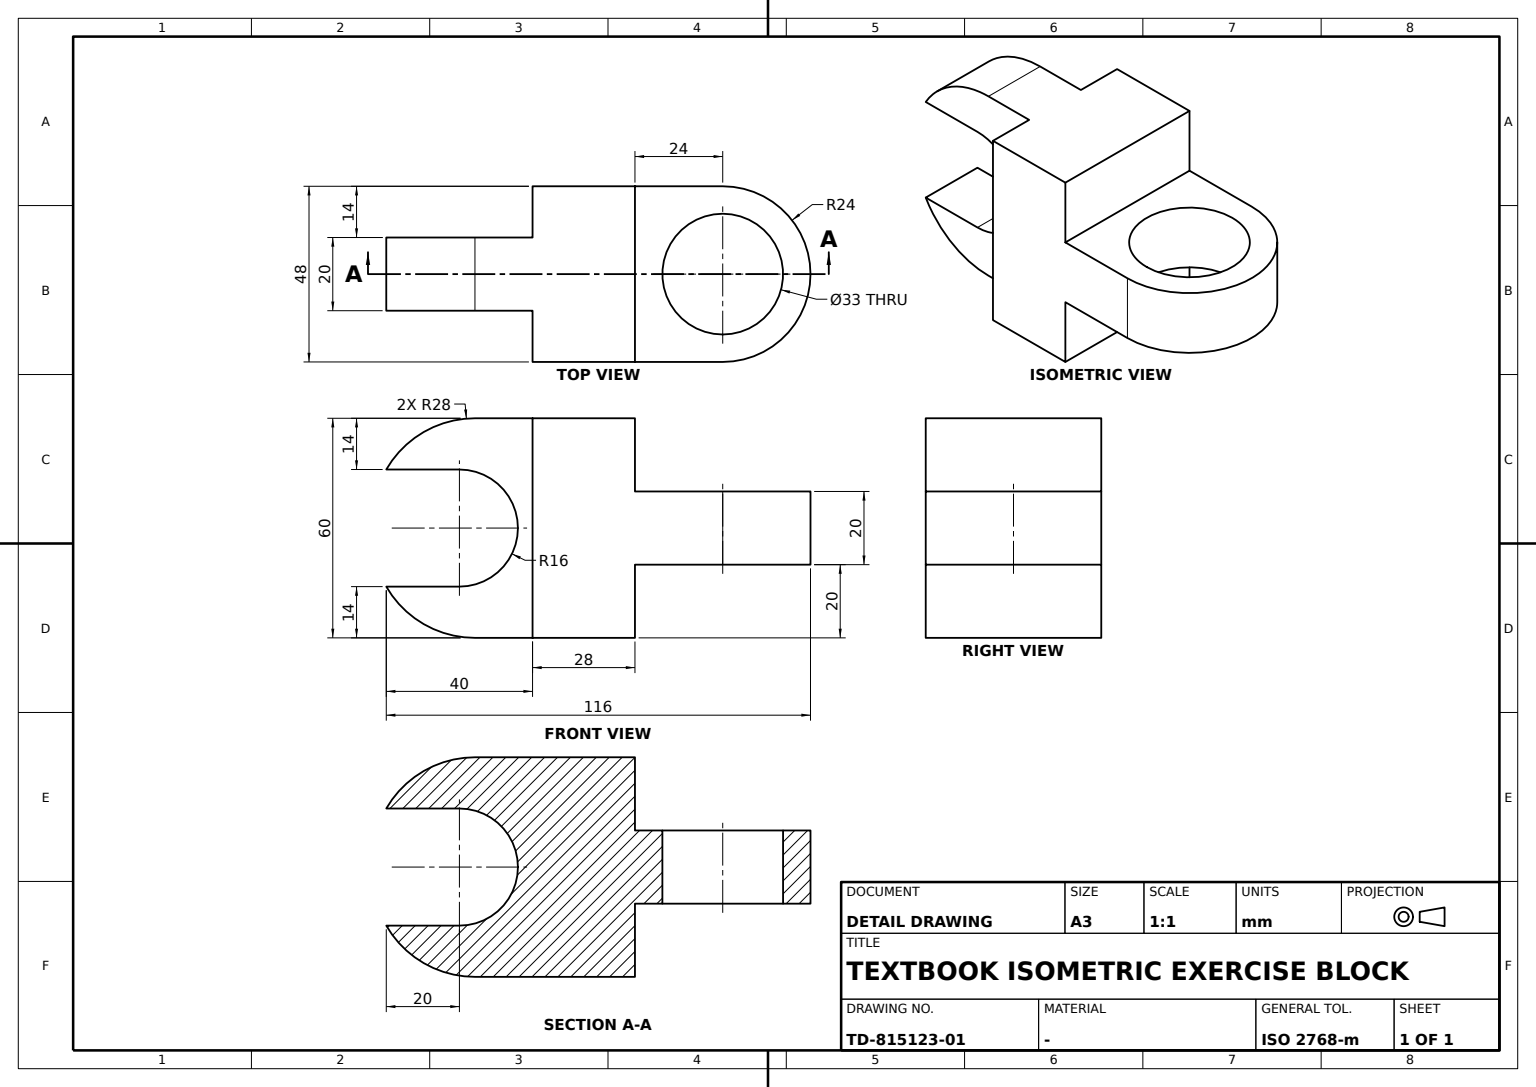
ISO-10303-21;
HEADER;
FILE_DESCRIPTION((''),'2;1');
FILE_NAME('','',(''),(''),'','','');
FILE_SCHEMA(('AUTOMOTIVE_DESIGN'));
ENDSEC;
DATA;
#1=APPLICATION_CONTEXT('');
#2=PRODUCT_CONTEXT('',#1,'mechanical');
#3=PRODUCT('','','',(#2));
#4=PRODUCT_DEFINITION_FORMATION('','',#3);
#5=PRODUCT_DEFINITION_CONTEXT('',#1,'design');
#6=PRODUCT_DEFINITION('','',#4,#5);
#7=PRODUCT_DEFINITION_SHAPE('','',#6);
#8=(LENGTH_UNIT()NAMED_UNIT(*)SI_UNIT(.MILLI.,.METRE.));
#9=(NAMED_UNIT(*)PLANE_ANGLE_UNIT()SI_UNIT($,.RADIAN.));
#10=(NAMED_UNIT(*)SI_UNIT($,.STERADIAN.)SOLID_ANGLE_UNIT());
#11=UNCERTAINTY_MEASURE_WITH_UNIT(LENGTH_MEASURE(1.E-05),#8,'distance_accuracy_value','');
#12=(GEOMETRIC_REPRESENTATION_CONTEXT(3)GLOBAL_UNCERTAINTY_ASSIGNED_CONTEXT((#11))GLOBAL_UNIT_ASSIGNED_CONTEXT((#8,#9,#10))REPRESENTATION_CONTEXT('',''));
#13=CARTESIAN_POINT('',(-10.,-18.,30.));
#14=VERTEX_POINT('',#13);
#15=CARTESIAN_POINT('',(-10.,-34.,14.));
#16=VERTEX_POINT('',#15);
#17=CARTESIAN_POINT('',(-10.,-34.,30.));
#18=DIRECTION('',(-1.,0.,0.));
#19=DIRECTION('',(0.,1.,0.));
#20=AXIS2_PLACEMENT_3D('',#17,#18,#19);
#21=CIRCLE('',#20,16.);
#22=EDGE_CURVE('',#14,#16,#21,.T.);
#23=ORIENTED_EDGE('',*,*,#22,.T.);
#24=CARTESIAN_POINT('',(10.,-34.,14.));
#25=VERTEX_POINT('',#24);
#26=CARTESIAN_POINT('',(-7.66,-34.,14.));
#27=VECTOR('',#18,1000.);
#28=LINE('',#26,#27);
#29=EDGE_CURVE('',#25,#16,#28,.T.);
#30=ORIENTED_EDGE('',*,*,#29,.F.);
#31=CARTESIAN_POINT('',(10.,-18.,30.));
#32=VERTEX_POINT('',#31);
#33=CARTESIAN_POINT('',(10.,-34.,30.));
#34=DIRECTION('',(1.,0.,0.));
#35=AXIS2_PLACEMENT_3D('',#33,#34,#19);
#36=CIRCLE('',#35,16.);
#37=EDGE_CURVE('',#25,#32,#36,.T.);
#38=ORIENTED_EDGE('',*,*,#37,.T.);
#39=CARTESIAN_POINT('',(-7.66,-18.,30.));
#40=LINE('',#39,#27);
#41=EDGE_CURVE('',#32,#14,#40,.T.);
#42=ORIENTED_EDGE('',*,*,#41,.T.);
#43=EDGE_LOOP('',(#23,#30,#38,#42));
#44=FACE_OUTER_BOUND('',#43,.T.);
#45=CARTESIAN_POINT('',(-7.66,-34.,30.));
#46=AXIS2_PLACEMENT_3D('',#45,#18,#19);
#47=CYLINDRICAL_SURFACE('',#46,16.);
#48=ADVANCED_FACE('',(#44),#47,.F.);
#49=CARTESIAN_POINT('',(-10.,-29.751289,60.));
#50=VERTEX_POINT('',#49);
#51=CARTESIAN_POINT('',(10.,-29.751289,60.));
#52=VERTEX_POINT('',#51);
#53=CARTESIAN_POINT('',(0.,-29.751289,60.));
#54=VECTOR('',#34,1000.);
#55=LINE('',#53,#54);
#56=EDGE_CURVE('',#50,#52,#55,.T.);
#57=ORIENTED_EDGE('',*,*,#56,.T.);
#58=CARTESIAN_POINT('',(10.,-14.,60.));
#59=VERTEX_POINT('',#58);
#60=CARTESIAN_POINT('',(10.,-21.875644,60.));
#61=DIRECTION('',(0.,-1.,0.));
#62=VECTOR('',#61,1000.);
#63=LINE('',#60,#62);
#64=EDGE_CURVE('',#59,#52,#63,.T.);
#65=ORIENTED_EDGE('',*,*,#64,.F.);
#66=CARTESIAN_POINT('',(-10.,-14.,60.));
#67=VERTEX_POINT('',#66);
#68=CARTESIAN_POINT('',(0.,-14.,60.));
#69=LINE('',#68,#54);
#70=EDGE_CURVE('',#67,#59,#69,.T.);
#71=ORIENTED_EDGE('',*,*,#70,.F.);
#72=CARTESIAN_POINT('',(-10.,-21.875644,60.));
#73=VECTOR('',#19,1000.);
#74=LINE('',#72,#73);
#75=EDGE_CURVE('',#50,#67,#74,.T.);
#76=ORIENTED_EDGE('',*,*,#75,.F.);
#77=EDGE_LOOP('',(#57,#65,#71,#76));
#78=FACE_OUTER_BOUND('',#77,.T.);
#79=CARTESIAN_POINT('',(0.,14.,60.));
#80=DIRECTION('',(0.,0.,1.));
#81=AXIS2_PLACEMENT_3D('',#79,#80,#61);
#82=PLANE('',#81);
#83=ADVANCED_FACE('',(#78),#82,.T.);
#84=CARTESIAN_POINT('',(24.,14.,40.));
#85=VERTEX_POINT('',#84);
#86=CARTESIAN_POINT('',(24.,14.,60.));
#87=VERTEX_POINT('',#86);
#88=CARTESIAN_POINT('',(24.,14.,50.));
#89=VECTOR('',#80,1000.);
#90=LINE('',#88,#89);
#91=EDGE_CURVE('',#85,#87,#90,.T.);
#92=ORIENTED_EDGE('',*,*,#91,.T.);
#93=CARTESIAN_POINT('',(24.,-14.,60.));
#94=VERTEX_POINT('',#93);
#95=CARTESIAN_POINT('',(24.,0.,60.));
#96=LINE('',#95,#62);
#97=EDGE_CURVE('',#87,#94,#96,.T.);
#98=ORIENTED_EDGE('',*,*,#97,.T.);
#99=CARTESIAN_POINT('',(24.,-14.,0.));
#100=VERTEX_POINT('',#99);
#101=CARTESIAN_POINT('',(24.,-14.,30.));
#102=DIRECTION('',(0.,0.,-1.));
#103=VECTOR('',#102,1000.);
#104=LINE('',#101,#103);
#105=EDGE_CURVE('',#94,#100,#104,.T.);
#106=ORIENTED_EDGE('',*,*,#105,.T.);
#107=CARTESIAN_POINT('',(24.,14.,0.));
#108=VERTEX_POINT('',#107);
#109=CARTESIAN_POINT('',(24.,0.,0.));
#110=LINE('',#109,#73);
#111=EDGE_CURVE('',#100,#108,#110,.T.);
#112=ORIENTED_EDGE('',*,*,#111,.T.);
#113=CARTESIAN_POINT('',(24.,14.,20.));
#114=VERTEX_POINT('',#113);
#115=CARTESIAN_POINT('',(24.,14.,10.));
#116=LINE('',#115,#89);
#117=EDGE_CURVE('',#108,#114,#116,.T.);
#118=ORIENTED_EDGE('',*,*,#117,.T.);
#119=CARTESIAN_POINT('',(24.,38.,20.));
#120=VERTEX_POINT('',#119);
#121=CARTESIAN_POINT('',(24.,26.,20.));
#122=LINE('',#121,#73);
#123=EDGE_CURVE('',#114,#120,#122,.T.);
#124=ORIENTED_EDGE('',*,*,#123,.T.);
#125=CARTESIAN_POINT('',(24.,38.,40.));
#126=VERTEX_POINT('',#125);
#127=CARTESIAN_POINT('',(24.,38.,30.));
#128=LINE('',#127,#89);
#129=EDGE_CURVE('',#120,#126,#128,.T.);
#130=ORIENTED_EDGE('',*,*,#129,.T.);
#131=CARTESIAN_POINT('',(24.,26.,40.));
#132=LINE('',#131,#62);
#133=EDGE_CURVE('',#126,#85,#132,.T.);
#134=ORIENTED_EDGE('',*,*,#133,.T.);
#135=EDGE_LOOP('',(#92,#98,#106,#112,#118,#124,#130,#134));
#136=FACE_OUTER_BOUND('',#135,.T.);
#137=AXIS2_PLACEMENT_3D('',#109,#34,#19);
#138=PLANE('',#137);
#139=ADVANCED_FACE('',(#136),#138,.T.);
#140=CARTESIAN_POINT('',(10.,-14.,0.));
#141=VERTEX_POINT('',#140);
#142=CARTESIAN_POINT('',(17.,-14.,0.));
#143=LINE('',#142,#54);
#144=EDGE_CURVE('',#141,#100,#143,.T.);
#145=ORIENTED_EDGE('',*,*,#144,.T.);
#146=ORIENTED_EDGE('',*,*,#105,.F.);
#147=CARTESIAN_POINT('',(17.,-14.,60.));
#148=LINE('',#147,#54);
#149=EDGE_CURVE('',#59,#94,#148,.T.);
#150=ORIENTED_EDGE('',*,*,#149,.F.);
#151=CARTESIAN_POINT('',(10.,-14.,30.));
#152=LINE('',#151,#103);
#153=EDGE_CURVE('',#59,#141,#152,.T.);
#154=ORIENTED_EDGE('',*,*,#153,.T.);
#155=EDGE_LOOP('',(#145,#146,#150,#154));
#156=FACE_OUTER_BOUND('',#155,.T.);
#157=AXIS2_PLACEMENT_3D('',#58,#19,#34);
#158=PLANE('',#157);
#159=ADVANCED_FACE('',(#156),#158,.F.);
#160=CARTESIAN_POINT('',(-24.,-14.,60.));
#161=VERTEX_POINT('',#160);
#162=CARTESIAN_POINT('',(-24.,-14.,0.));
#163=VERTEX_POINT('',#162);
#164=CARTESIAN_POINT('',(-24.,-14.,30.));
#165=LINE('',#164,#103);
#166=EDGE_CURVE('',#161,#163,#165,.T.);
#167=ORIENTED_EDGE('',*,*,#166,.F.);
#168=CARTESIAN_POINT('',(-24.,14.,60.));
#169=VERTEX_POINT('',#168);
#170=CARTESIAN_POINT('',(-24.,0.,60.));
#171=LINE('',#170,#62);
#172=EDGE_CURVE('',#169,#161,#171,.T.);
#173=ORIENTED_EDGE('',*,*,#172,.F.);
#174=CARTESIAN_POINT('',(-24.,14.,40.));
#175=VERTEX_POINT('',#174);
#176=CARTESIAN_POINT('',(-24.,14.,50.));
#177=LINE('',#176,#89);
#178=EDGE_CURVE('',#175,#169,#177,.T.);
#179=ORIENTED_EDGE('',*,*,#178,.F.);
#180=CARTESIAN_POINT('',(-24.,38.,40.));
#181=VERTEX_POINT('',#180);
#182=CARTESIAN_POINT('',(-24.,26.,40.));
#183=LINE('',#182,#62);
#184=EDGE_CURVE('',#181,#175,#183,.T.);
#185=ORIENTED_EDGE('',*,*,#184,.F.);
#186=CARTESIAN_POINT('',(-24.,38.,20.));
#187=VERTEX_POINT('',#186);
#188=CARTESIAN_POINT('',(-24.,38.,30.));
#189=LINE('',#188,#89);
#190=EDGE_CURVE('',#187,#181,#189,.T.);
#191=ORIENTED_EDGE('',*,*,#190,.F.);
#192=CARTESIAN_POINT('',(-24.,14.,20.));
#193=VERTEX_POINT('',#192);
#194=CARTESIAN_POINT('',(-24.,26.,20.));
#195=LINE('',#194,#73);
#196=EDGE_CURVE('',#193,#187,#195,.T.);
#197=ORIENTED_EDGE('',*,*,#196,.F.);
#198=CARTESIAN_POINT('',(-24.,14.,0.));
#199=VERTEX_POINT('',#198);
#200=CARTESIAN_POINT('',(-24.,14.,10.));
#201=LINE('',#200,#89);
#202=EDGE_CURVE('',#199,#193,#201,.T.);
#203=ORIENTED_EDGE('',*,*,#202,.F.);
#204=CARTESIAN_POINT('',(-24.,0.,0.));
#205=LINE('',#204,#73);
#206=EDGE_CURVE('',#163,#199,#205,.T.);
#207=ORIENTED_EDGE('',*,*,#206,.F.);
#208=EDGE_LOOP('',(#167,#173,#179,#185,#191,#197,#203,#207));
#209=FACE_OUTER_BOUND('',#208,.T.);
#210=AXIS2_PLACEMENT_3D('',#204,#34,#19);
#211=PLANE('',#210);
#212=ADVANCED_FACE('',(#209),#211,.F.);
#213=CARTESIAN_POINT('',(10.,-34.,46.));
#214=VERTEX_POINT('',#213);
#215=EDGE_CURVE('',#32,#214,#36,.T.);
#216=ORIENTED_EDGE('',*,*,#215,.F.);
#217=ORIENTED_EDGE('',*,*,#37,.F.);
#218=CARTESIAN_POINT('',(10.,-54.,14.));
#219=VERTEX_POINT('',#218);
#220=CARTESIAN_POINT('',(10.,-44.,14.));
#221=LINE('',#220,#73);
#222=EDGE_CURVE('',#219,#25,#221,.T.);
#223=ORIENTED_EDGE('',*,*,#222,.F.);
#224=CARTESIAN_POINT('',(10.,-29.751289,0.));
#225=VERTEX_POINT('',#224);
#226=CARTESIAN_POINT('',(10.,-29.751289,28.));
#227=AXIS2_PLACEMENT_3D('',#226,#18,#61);
#228=CIRCLE('',#227,28.);
#229=EDGE_CURVE('',#225,#219,#228,.T.);
#230=ORIENTED_EDGE('',*,*,#229,.F.);
#231=CARTESIAN_POINT('',(10.,-21.875644,0.));
#232=LINE('',#231,#62);
#233=EDGE_CURVE('',#141,#225,#232,.T.);
#234=ORIENTED_EDGE('',*,*,#233,.F.);
#235=ORIENTED_EDGE('',*,*,#153,.F.);
#236=ORIENTED_EDGE('',*,*,#64,.T.);
#237=CARTESIAN_POINT('',(10.,-54.,46.));
#238=VERTEX_POINT('',#237);
#239=CARTESIAN_POINT('',(10.,-29.751289,32.));
#240=AXIS2_PLACEMENT_3D('',#239,#18,#61);
#241=CIRCLE('',#240,28.);
#242=EDGE_CURVE('',#238,#52,#241,.T.);
#243=ORIENTED_EDGE('',*,*,#242,.F.);
#244=CARTESIAN_POINT('',(10.,-44.,46.));
#245=LINE('',#244,#62);
#246=EDGE_CURVE('',#214,#238,#245,.T.);
#247=ORIENTED_EDGE('',*,*,#246,.F.);
#248=EDGE_LOOP('',(#216,#217,#223,#230,#234,#235,#236,#243,#247));
#249=FACE_OUTER_BOUND('',#248,.T.);
#250=AXIS2_PLACEMENT_3D('',#58,#34,#61);
#251=PLANE('',#250);
#252=ADVANCED_FACE('',(#249),#251,.T.);
#253=ORIENTED_EDGE('',*,*,#144,.F.);
#254=CARTESIAN_POINT('',(-10.,-14.,0.));
#255=VERTEX_POINT('',#254);
#256=CARTESIAN_POINT('',(0.,-14.,0.));
#257=LINE('',#256,#54);
#258=EDGE_CURVE('',#255,#141,#257,.T.);
#259=ORIENTED_EDGE('',*,*,#258,.F.);
#260=CARTESIAN_POINT('',(-17.,-14.,0.));
#261=LINE('',#260,#54);
#262=EDGE_CURVE('',#163,#255,#261,.T.);
#263=ORIENTED_EDGE('',*,*,#262,.F.);
#264=ORIENTED_EDGE('',*,*,#206,.T.);
#265=CARTESIAN_POINT('',(0.,14.,0.));
#266=LINE('',#265,#54);
#267=EDGE_CURVE('',#199,#108,#266,.T.);
#268=ORIENTED_EDGE('',*,*,#267,.T.);
#269=ORIENTED_EDGE('',*,*,#111,.F.);
#270=EDGE_LOOP('',(#253,#259,#263,#264,#268,#269));
#271=FACE_OUTER_BOUND('',#270,.T.);
#272=AXIS2_PLACEMENT_3D('',#256,#102,#19);
#273=PLANE('',#272);
#274=ADVANCED_FACE('',(#271),#273,.T.);
#275=ORIENTED_EDGE('',*,*,#202,.T.);
#276=CARTESIAN_POINT('',(0.,14.,20.));
#277=LINE('',#276,#54);
#278=EDGE_CURVE('',#193,#114,#277,.T.);
#279=ORIENTED_EDGE('',*,*,#278,.T.);
#280=ORIENTED_EDGE('',*,*,#117,.F.);
#281=ORIENTED_EDGE('',*,*,#267,.F.);
#282=EDGE_LOOP('',(#275,#279,#280,#281));
#283=FACE_OUTER_BOUND('',#282,.T.);
#284=AXIS2_PLACEMENT_3D('',#265,#19,#80);
#285=PLANE('',#284);
#286=ADVANCED_FACE('',(#283),#285,.T.);
#287=CARTESIAN_POINT('',(-10.,-54.,14.));
#288=VERTEX_POINT('',#287);
#289=CARTESIAN_POINT('',(-10.,-44.,14.));
#290=LINE('',#289,#73);
#291=EDGE_CURVE('',#288,#16,#290,.T.);
#292=ORIENTED_EDGE('',*,*,#291,.F.);
#293=CARTESIAN_POINT('',(0.,-54.,14.));
#294=LINE('',#293,#54);
#295=EDGE_CURVE('',#288,#219,#294,.T.);
#296=ORIENTED_EDGE('',*,*,#295,.T.);
#297=ORIENTED_EDGE('',*,*,#222,.T.);
#298=ORIENTED_EDGE('',*,*,#29,.T.);
#299=EDGE_LOOP('',(#292,#296,#297,#298));
#300=FACE_OUTER_BOUND('',#299,.T.);
#301=AXIS2_PLACEMENT_3D('',#218,#80,#19);
#302=PLANE('',#301);
#303=ADVANCED_FACE('',(#300),#302,.T.);
#304=CARTESIAN_POINT('',(-16.5,38.,40.));
#305=VERTEX_POINT('',#304);
#306=CARTESIAN_POINT('',(16.5,38.,40.));
#307=VERTEX_POINT('',#306);
#308=CARTESIAN_POINT('',(0.,38.,40.));
#309=AXIS2_PLACEMENT_3D('',#308,#80,#34);
#310=CIRCLE('',#309,16.5);
#311=EDGE_CURVE('',#305,#307,#310,.T.);
#312=ORIENTED_EDGE('',*,*,#311,.T.);
#313=CARTESIAN_POINT('',(16.5,38.,20.));
#314=VERTEX_POINT('',#313);
#315=CARTESIAN_POINT('',(16.5,38.,19.34));
#316=LINE('',#315,#103);
#317=EDGE_CURVE('',#307,#314,#316,.T.);
#318=ORIENTED_EDGE('',*,*,#317,.T.);
#319=CARTESIAN_POINT('',(-16.5,38.,20.));
#320=VERTEX_POINT('',#319);
#321=CARTESIAN_POINT('',(0.,38.,20.));
#322=AXIS2_PLACEMENT_3D('',#321,#102,#19);
#323=CIRCLE('',#322,16.5);
#324=EDGE_CURVE('',#314,#320,#323,.T.);
#325=ORIENTED_EDGE('',*,*,#324,.T.);
#326=CARTESIAN_POINT('',(-16.5,38.,19.34));
#327=LINE('',#326,#103);
#328=EDGE_CURVE('',#305,#320,#327,.T.);
#329=ORIENTED_EDGE('',*,*,#328,.F.);
#330=EDGE_LOOP('',(#312,#318,#325,#329));
#331=FACE_OUTER_BOUND('',#330,.T.);
#332=CARTESIAN_POINT('',(0.,38.,19.34));
#333=AXIS2_PLACEMENT_3D('',#332,#102,#34);
#334=CYLINDRICAL_SURFACE('',#333,16.5);
#335=ADVANCED_FACE('',(#331),#334,.F.);
#336=CARTESIAN_POINT('',(-10.,-29.751289,0.));
#337=VERTEX_POINT('',#336);
#338=CARTESIAN_POINT('',(-10.,-21.875644,0.));
#339=LINE('',#338,#62);
#340=EDGE_CURVE('',#255,#337,#339,.T.);
#341=ORIENTED_EDGE('',*,*,#340,.T.);
#342=CARTESIAN_POINT('',(-10.,-29.751289,28.));
#343=AXIS2_PLACEMENT_3D('',#342,#34,#19);
#344=CIRCLE('',#343,28.);
#345=EDGE_CURVE('',#288,#337,#344,.T.);
#346=ORIENTED_EDGE('',*,*,#345,.F.);
#347=ORIENTED_EDGE('',*,*,#291,.T.);
#348=ORIENTED_EDGE('',*,*,#22,.F.);
#349=CARTESIAN_POINT('',(-10.,-34.,46.));
#350=VERTEX_POINT('',#349);
#351=EDGE_CURVE('',#350,#14,#21,.T.);
#352=ORIENTED_EDGE('',*,*,#351,.F.);
#353=CARTESIAN_POINT('',(-10.,-54.,46.));
#354=VERTEX_POINT('',#353);
#355=CARTESIAN_POINT('',(-10.,-44.,46.));
#356=LINE('',#355,#73);
#357=EDGE_CURVE('',#354,#350,#356,.T.);
#358=ORIENTED_EDGE('',*,*,#357,.F.);
#359=CARTESIAN_POINT('',(-10.,-29.751289,32.));
#360=AXIS2_PLACEMENT_3D('',#359,#34,#19);
#361=CIRCLE('',#360,28.);
#362=EDGE_CURVE('',#50,#354,#361,.T.);
#363=ORIENTED_EDGE('',*,*,#362,.F.);
#364=ORIENTED_EDGE('',*,*,#75,.T.);
#365=CARTESIAN_POINT('',(-10.,-14.,30.));
#366=LINE('',#365,#103);
#367=EDGE_CURVE('',#67,#255,#366,.T.);
#368=ORIENTED_EDGE('',*,*,#367,.T.);
#369=EDGE_LOOP('',(#341,#346,#347,#348,#352,#358,#363,#364,#368));
#370=FACE_OUTER_BOUND('',#369,.T.);
#371=CARTESIAN_POINT('',(-10.,-58.719479,60.));
#372=AXIS2_PLACEMENT_3D('',#371,#18,#19);
#373=PLANE('',#372);
#374=ADVANCED_FACE('',(#370),#373,.T.);
#375=CARTESIAN_POINT('',(0.,-54.,46.));
#376=LINE('',#375,#54);
#377=EDGE_CURVE('',#354,#238,#376,.T.);
#378=ORIENTED_EDGE('',*,*,#377,.T.);
#379=ORIENTED_EDGE('',*,*,#242,.T.);
#380=ORIENTED_EDGE('',*,*,#56,.F.);
#381=ORIENTED_EDGE('',*,*,#362,.T.);
#382=EDGE_LOOP('',(#378,#379,#380,#381));
#383=FACE_OUTER_BOUND('',#382,.T.);
#384=CARTESIAN_POINT('',(0.,-29.751289,32.));
#385=DIRECTION('',(0.,-0.866025404,0.5));
#386=AXIS2_PLACEMENT_3D('',#384,#34,#385);
#387=CYLINDRICAL_SURFACE('',#386,28.);
#388=ADVANCED_FACE('',(#383),#387,.T.);
#389=CARTESIAN_POINT('',(-7.66,-34.,46.));
#390=LINE('',#389,#27);
#391=EDGE_CURVE('',#214,#350,#390,.T.);
#392=ORIENTED_EDGE('',*,*,#391,.F.);
#393=ORIENTED_EDGE('',*,*,#246,.T.);
#394=ORIENTED_EDGE('',*,*,#377,.F.);
#395=ORIENTED_EDGE('',*,*,#357,.T.);
#396=EDGE_LOOP('',(#392,#393,#394,#395));
#397=FACE_OUTER_BOUND('',#396,.T.);
#398=AXIS2_PLACEMENT_3D('',#237,#80,#19);
#399=PLANE('',#398);
#400=ADVANCED_FACE('',(#397),#399,.F.);
#401=ORIENTED_EDGE('',*,*,#317,.F.);
#402=EDGE_CURVE('',#307,#305,#310,.T.);
#403=ORIENTED_EDGE('',*,*,#402,.T.);
#404=ORIENTED_EDGE('',*,*,#328,.T.);
#405=EDGE_CURVE('',#320,#314,#323,.T.);
#406=ORIENTED_EDGE('',*,*,#405,.T.);
#407=EDGE_LOOP('',(#401,#403,#404,#406));
#408=FACE_OUTER_BOUND('',#407,.T.);
#409=ADVANCED_FACE('',(#408),#334,.F.);
#410=CARTESIAN_POINT('',(0.,14.,40.));
#411=LINE('',#410,#54);
#412=EDGE_CURVE('',#175,#85,#411,.T.);
#413=ORIENTED_EDGE('',*,*,#412,.F.);
#414=ORIENTED_EDGE('',*,*,#178,.T.);
#415=LINE('',#79,#54);
#416=EDGE_CURVE('',#169,#87,#415,.T.);
#417=ORIENTED_EDGE('',*,*,#416,.T.);
#418=ORIENTED_EDGE('',*,*,#91,.F.);
#419=EDGE_LOOP('',(#413,#414,#417,#418));
#420=FACE_OUTER_BOUND('',#419,.T.);
#421=ADVANCED_FACE('',(#420),#285,.T.);
#422=ORIENTED_EDGE('',*,*,#340,.F.);
#423=ORIENTED_EDGE('',*,*,#258,.T.);
#424=ORIENTED_EDGE('',*,*,#233,.T.);
#425=CARTESIAN_POINT('',(0.,-29.751289,0.));
#426=LINE('',#425,#54);
#427=EDGE_CURVE('',#337,#225,#426,.T.);
#428=ORIENTED_EDGE('',*,*,#427,.F.);
#429=EDGE_LOOP('',(#422,#423,#424,#428));
#430=FACE_OUTER_BOUND('',#429,.T.);
#431=ADVANCED_FACE('',(#430),#273,.T.);
#432=ORIENTED_EDGE('',*,*,#70,.T.);
#433=ORIENTED_EDGE('',*,*,#149,.T.);
#434=ORIENTED_EDGE('',*,*,#97,.F.);
#435=ORIENTED_EDGE('',*,*,#416,.F.);
#436=ORIENTED_EDGE('',*,*,#172,.T.);
#437=CARTESIAN_POINT('',(-17.,-14.,60.));
#438=LINE('',#437,#54);
#439=EDGE_CURVE('',#161,#67,#438,.T.);
#440=ORIENTED_EDGE('',*,*,#439,.T.);
#441=EDGE_LOOP('',(#432,#433,#434,#435,#436,#440));
#442=FACE_OUTER_BOUND('',#441,.T.);
#443=ADVANCED_FACE('',(#442),#82,.T.);
#444=AXIS2_PLACEMENT_3D('',#321,#80,#19);
#445=CIRCLE('',#444,24.);
#446=EDGE_CURVE('',#120,#187,#445,.T.);
#447=ORIENTED_EDGE('',*,*,#446,.T.);
#448=ORIENTED_EDGE('',*,*,#190,.T.);
#449=AXIS2_PLACEMENT_3D('',#308,#102,#61);
#450=CIRCLE('',#449,24.);
#451=EDGE_CURVE('',#181,#126,#450,.T.);
#452=ORIENTED_EDGE('',*,*,#451,.T.);
#453=ORIENTED_EDGE('',*,*,#129,.F.);
#454=EDGE_LOOP('',(#447,#448,#452,#453));
#455=FACE_OUTER_BOUND('',#454,.T.);
#456=CARTESIAN_POINT('',(0.,38.,30.));
#457=AXIS2_PLACEMENT_3D('',#456,#102,#18);
#458=CYLINDRICAL_SURFACE('',#457,24.);
#459=ADVANCED_FACE('',(#455),#458,.T.);
#460=ORIENTED_EDGE('',*,*,#391,.T.);
#461=ORIENTED_EDGE('',*,*,#351,.T.);
#462=ORIENTED_EDGE('',*,*,#41,.F.);
#463=ORIENTED_EDGE('',*,*,#215,.T.);
#464=EDGE_LOOP('',(#460,#461,#462,#463));
#465=FACE_OUTER_BOUND('',#464,.T.);
#466=ADVANCED_FACE('',(#465),#47,.F.);
#467=ORIENTED_EDGE('',*,*,#427,.T.);
#468=ORIENTED_EDGE('',*,*,#229,.T.);
#469=ORIENTED_EDGE('',*,*,#295,.F.);
#470=ORIENTED_EDGE('',*,*,#345,.T.);
#471=EDGE_LOOP('',(#467,#468,#469,#470));
#472=FACE_OUTER_BOUND('',#471,.T.);
#473=CARTESIAN_POINT('',(0.,-29.751289,28.));
#474=DIRECTION('',(0.,-0.866025404,-0.5));
#475=AXIS2_PLACEMENT_3D('',#473,#18,#474);
#476=CYLINDRICAL_SURFACE('',#475,28.);
#477=ADVANCED_FACE('',(#472),#476,.T.);
#478=ORIENTED_EDGE('',*,*,#262,.T.);
#479=ORIENTED_EDGE('',*,*,#367,.F.);
#480=ORIENTED_EDGE('',*,*,#439,.F.);
#481=ORIENTED_EDGE('',*,*,#166,.T.);
#482=EDGE_LOOP('',(#478,#479,#480,#481));
#483=FACE_OUTER_BOUND('',#482,.T.);
#484=ADVANCED_FACE('',(#483),#158,.F.);
#485=ORIENTED_EDGE('',*,*,#412,.T.);
#486=ORIENTED_EDGE('',*,*,#133,.F.);
#487=ORIENTED_EDGE('',*,*,#451,.F.);
#488=ORIENTED_EDGE('',*,*,#184,.T.);
#489=EDGE_LOOP('',(#485,#486,#487,#488));
#490=FACE_OUTER_BOUND('',#489,.T.);
#491=ORIENTED_EDGE('',*,*,#402,.F.);
#492=ORIENTED_EDGE('',*,*,#311,.F.);
#493=EDGE_LOOP('',(#491,#492));
#494=FACE_BOUND('',#493,.T.);
#495=CARTESIAN_POINT('',(0.,62.,40.));
#496=AXIS2_PLACEMENT_3D('',#495,#80,#61);
#497=PLANE('',#496);
#498=ADVANCED_FACE('',(#490,#494),#497,.T.);
#499=ORIENTED_EDGE('',*,*,#278,.F.);
#500=ORIENTED_EDGE('',*,*,#196,.T.);
#501=ORIENTED_EDGE('',*,*,#446,.F.);
#502=ORIENTED_EDGE('',*,*,#123,.F.);
#503=EDGE_LOOP('',(#499,#500,#501,#502));
#504=FACE_OUTER_BOUND('',#503,.T.);
#505=ORIENTED_EDGE('',*,*,#405,.F.);
#506=ORIENTED_EDGE('',*,*,#324,.F.);
#507=EDGE_LOOP('',(#505,#506));
#508=FACE_BOUND('',#507,.T.);
#509=AXIS2_PLACEMENT_3D('',#276,#102,#19);
#510=PLANE('',#509);
#511=ADVANCED_FACE('',(#504,#508),#510,.T.);
#512=CLOSED_SHELL('',(#48,#83,#139,#159,#212,#252,#274,#286,#303,#335,#374,#388,#400,#409,#421,#431,#443,#459,#466,#477,#484,#498,#511));
#513=MANIFOLD_SOLID_BREP('',#512);
#514=ADVANCED_BREP_SHAPE_REPRESENTATION('',(#513),#12);
#515=SHAPE_DEFINITION_REPRESENTATION(#7,#514);
ENDSEC;
END-ISO-10303-21;
